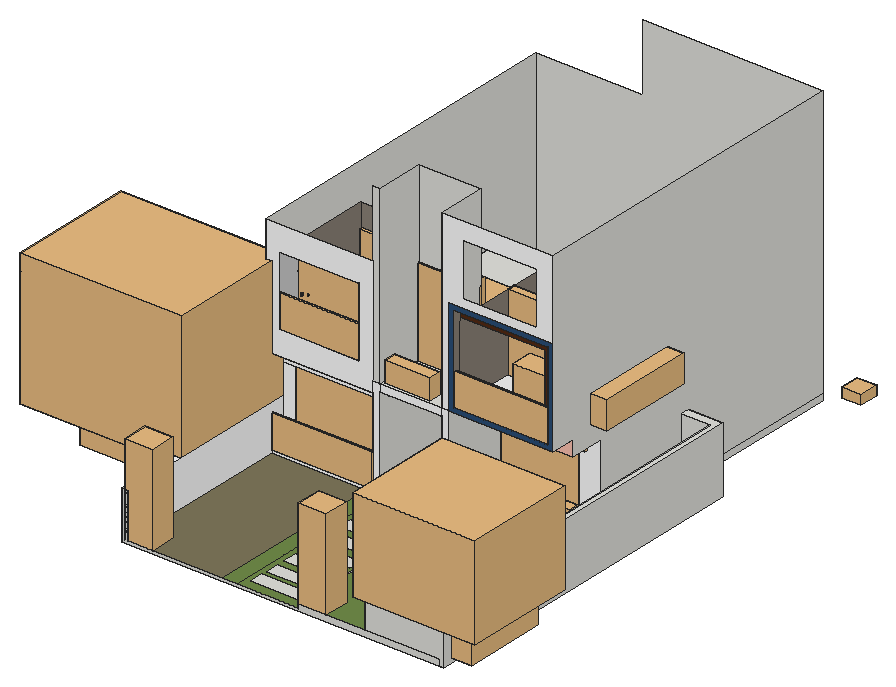
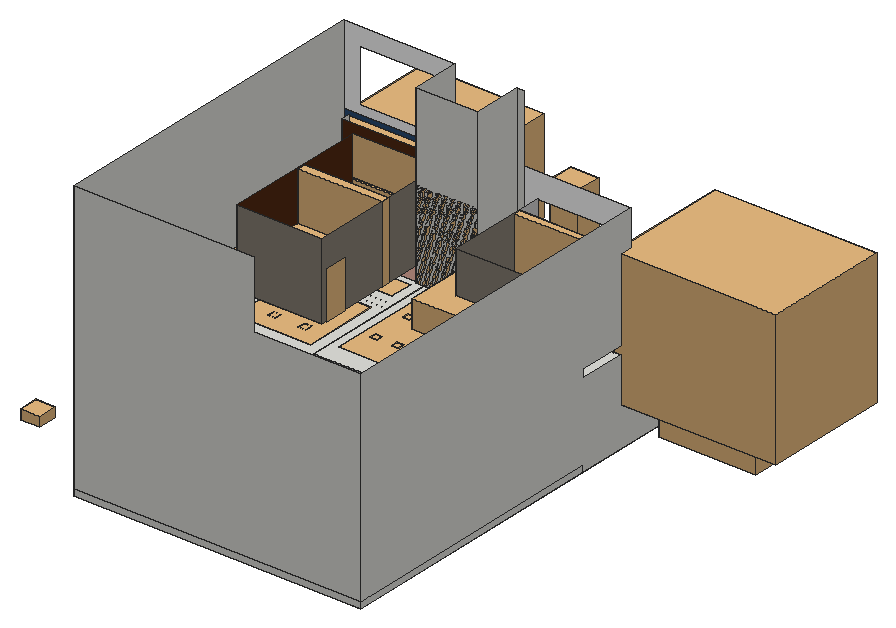
# SketchUp Ruby script. Lengths in inches.
U = 1.inch
M = Sketchup.active_model
def pt(a) = Geom::Point3d.new(a.map { |v| v * U })
def face(e, loops, mat)
  f = e.add_face(loops[0].map { |a| pt(a) })
  loops[1..].each { |l| e.add_face(l.map { |a| pt(a) }).erase! }
  f.material = f.back_material = mat if mat
  f
end
# faces: each face lists its corners as indices into pts; further lists are holes
def faces(e, pts, list, mat = nil) = list.each { |f| face(e, (f[0].is_a?(Array) ? f : [f]).map { |l| l.map { |i| pts[i] } }, mat) }
# xy, xz, yz: faces in a plane at the given z, y or x. An outline is a flat list of corners, or four numbers for a rectangle; further outlines are holes
def ring(l) = l.size == 4 ? [[l[0], l[1]], [l[2], l[1]], [l[2], l[3]], [l[0], l[3]]] : l.each_slice(2).to_a
def flat(e, list, mat, &to3) = list.each { |f| face(e, (f[0].is_a?(Array) ? f : [f]).map { |l| ring(l).map { |u, v| to3.(u, v) } }, mat) }
def xy(e, z, list, mat = nil) = flat(e, list, mat) { |x, y| [x, y, z] }
def xz(e, y, list, mat = nil) = flat(e, list, mat) { |x, z| [x, y, z] }
def yz(e, x, list, mat = nil) = flat(e, list, mat) { |y, z| [x, y, z] }
def lines(e, pts, list) = list.each { |a, b| e.add_line(pt(pts[a]), pt(pts[b])) }
# prism: a flat outline (further loops are holes) pulled along v
def prism(e, loops, v, mat = nil)
  f = face(e, loops, mat); d = Geom::Vector3d.new(v.map { |x| x * U })
  f.pushpull(f.normal.samedirection?(d) ? d.length : -d.length)
end
def box(e, o, s, mat = nil) = prism(e, [[o, [o[0] + s[0], o[1], o[2]], [o[0] + s[0], o[1] + s[1], o[2]], [o[0], o[1] + s[1], o[2]]]], [0, 0, s[2]], mat)
def at(x, y, z, deg = 0) = Geom::Transformation.translation(pt([x, y, z])) * Geom::Transformation.rotation(ORIGIN, Z_AXIS, deg.degrees)
def axes(o, x, y, z) = Geom::Transformation.new([*x, 0, *y, 0, *z, 0, *pt(o).to_a, 1])
def part(name) = M.definitions.add(name)
# library, detail: a bought-in or finely detailed component or shape, given as its bounding box
def library(name, o, s) = part(name).tap { |d| box(d.entities, o, s) }
def detail(e, o, s) = box(e.add_group.entities, o, s)
def put(e, d, t, mat = nil) = e.add_instance(d, t).tap { |i| i.material = mat if mat }
def group(e, t, mat = nil) = e.add_group.tap { |g| g.transformation = t; g.material = mat if mat }.entities
root = M.entities
M.materials.add("AM113_062_Tilia").color = [58, 81, 37]
M.materials.add("AM113_062_Tilia_Bark").color = [88, 85, 72]
M.materials.add("Concrete White 02 100cm").color = [209, 209, 209]
M.materials.add("Grass D 200cm").color = [112, 140, 73]
M.materials.add("Gravel E01 80cm").color = [127, 119, 91]
M.materials.add("Heather_Band").color = [140, 131, 120]
M.materials.add("Heather_PantShadow").color = [42, 79, 119]
M.materials.add("Tiles Marble Black 01 160cm").color = [31, 31, 31]
M.materials.add("Tiles Marble White 03 180cm").color = [241, 241, 241]
M.materials.add("Wall Paint White Semigloss 300cm").color = [255, 255, 255]
M.materials.add("Wood Mahogany 33-46 100cm").color = [83, 42, 20]
M.materials.add("[0131_Silver]").color = [192, 192, 192]
M.materials.add("[Color B01]").color = [255, 196, 178]
M.materials.add("efeu1").color = [18, 25, 13]
M.materials.add("efeu2").color = [43, 57, 29]
c1 = library("Lamp Outdoor 94-18",[-17.37,-12.57,0.01],[34.74,31.82,112.44])
c2 = library("skp108",[-1.77,-1.13,-0.05],[3.15,2.48,2.06])
c3 = library("skp10A",[-2.51,-1.55,0.73],[4.12,3.36,1.8])
c4 = part("tree")
put(c4.entities,c2,axes([-3.75,5.02,4.3],[-100,0,0],[0,100,0],[0,0,100]))
put(c4.entities,c3,axes([-24.21,-1.17,-13.42],[-100,0,0],[0,100,0],[0,0,100]))
c5 = library("Group\#39",[0,0,0],[56.8,25.91,35.15])
c6 = library("Rossi Sofa",[-52.17,-19.09,0],[104.34,38.18,34.45])
c7 = library("AM113_062_Tilia_Defintion",[-350.67,-364.73,-2.58],[672.29,726.36,1000])
c8 = library("AM113_062_Tilia_Defintion1",[-524.84,-500,219.37],[933.41,1000,877.77])
c9 = part("Group4\#1")
put(c9.entities,c7,axes([0,0,0],[0.28109,0,0],[0,0.28109,0],[0,0,0.28109]),"AM113_062_Tilia_Bark")
put(c9.entities,c8,axes([0,0,0],[0.33697,0,0],[0,0.33697,0],[0,0,0.33697]),"AM113_062_Tilia")
c10 = library("Group\#41",[0,0,0],[116.43,13.29,95.4])
c11 = library("My+Glass_Railing\#2",[-0.08,0,0],[125.4,2.52,40.9])
c12 = library("Entrance door assembly",[0,0,0],[51.57,9.61,84.84])
c13 = library("Dome Light",[-12,-12,0],[24,24,12])
c14 = part("Tlon Cubo 860 Ceiling 152 005")
xy(c14.entities,-3.04,[[-16.54,-16.54,-16.54,16.54,16.54,-16.54],[16.54,-16.54,-16.54,16.54,16.54,16.54]])
xy(c14.entities,0,[[-16.93,-16.93,16.93,-16.93,-16.93,16.93],[16.93,-16.93,16.93,16.93,-16.93,16.93]])
xz(c14.entities,-16.93,[[-16.93,-3.79,16.93,-3.79,-16.93,0],[16.93,-3.79,16.93,0,-16.93,0]])
xz(c14.entities,-16.3,[[-16.3,-3.66,-16.3,-3.24,16.3,-3.24],[-16.3,-3.66,16.3,-3.24,16.3,-3.66]])
xz(c14.entities,16.3,[[-16.3,-3.66,16.3,-3.24,-16.3,-3.24],[-16.3,-3.66,16.3,-3.66,16.3,-3.24]])
xz(c14.entities,16.93,[[-16.93,-3.79,-16.93,0,16.93,0],[-16.93,-3.79,16.93,0,16.93,-3.79]])
yz(c14.entities,-16.93,[[-16.93,-3.79,-16.93,0,16.93,0],[-16.93,-3.79,16.93,0,16.93,-3.79]])
yz(c14.entities,-16.3,[[-16.3,-3.66,16.3,-3.66,-16.3,-3.24],[16.3,-3.66,16.3,-3.24,-16.3,-3.24]])
yz(c14.entities,16.3,[[-16.3,-3.66,-16.3,-3.24,16.3,-3.66],[16.3,-3.66,-16.3,-3.24,16.3,-3.24]])
yz(c14.entities,16.93,[[-16.93,-3.79,16.93,-3.79,-16.93,0],[16.93,-3.79,16.93,0,-16.93,0]])
p = [[-16.93,-16.93,-3.79],[-16.93,16.93,-3.79],[-16.3,16.3,-3.66],[-16.3,-16.3,-3.66],[16.93,-16.93,-3.79],[16.3,-16.3,-3.66],
  [16.93,16.93,-3.79],[16.3,16.3,-3.66]]
faces(c14.entities,p,[[0,1,2],[2,3,0],[4,0,3],[3,5,4],[6,4,5],[5,7,6],[2,1,6],[6,7,2]])
c15 = library("Mesh Light\#3",[-0.5,-0.5,-0.1],[1,1,0.2])
c16 = library("Lamp Ceiling 114-44",[-1.26,-1.26,-3.9375],[2.52,2.52,3.9375])
c17 = library("Tlon Light 450 Ceiling 152 006",[-8.86,-8.86,-3.78],[17.72,17.72,3.56])
c18 = library("Group\#10",[-0.5,-0.5,-0.1],[94.5625,94.5625,0.2])
c19 = library("Group\#15",[-0.5,-0.5,-0.1],[105.0625,28.875,0.2])
c20 = library("Group\#9",[-0.5,-0.5,-0.1],[56.6875,175.375,0.2])
c21 = library("Planted timber trough",[0,0,0],[56.02,15.3,25.28])
c22 = library("Wall Panel 104-26",[-34.24,-2.8,0],[68.48,2.8,108.01])
c23 = library("Door 243 067",[-20.85,-3,0],[41.7,6,82.46])
c24 = library("BED_01",[-66.74,-61.37,0],[192.98,188.94,55.24])
c25 = library("My+Glass_Railing",[-0.08,0,0],[117.37,2.52,40.9])
c26 = library("My+Glass_Railing\#1",[-0.0625,0,0],[99.04,2.52,40.9])
c27 = part("ivyleaf_10")
p = [[0,0.5,-0.03],[-0.0625,2.02,-0.43],[-0.19,2.01,-0.46],[-0.54,1.05,-0.29],[-0.52,0.625,-0.18],[-0.83,0.76,-0.28],
  [-1.16,0.64,-0.33],[-1.15,0.33,-0.24],[-0.77,-0.39,0.02],[-0.3,-0.51,0.16],[0.04,-0.48,0.23],[-0.02,2.01,-0.4375],
  [-0.06,2.01,-0.43],[0.04,-0.49,0.23],[0.67,-0.49,0.14],[1.38,0.36,-0.2],[1.375,0.51,-0.24],[0.81,0.65,-0.19],
  [0.62,0.59,-0.15],[0.6,1.09,-0.28],[0.5,1.23,-0.31]]
faces(c27.entities,p,[[0,1,2,3,4,5,6,7,8,9,10],[11,12,0,13,14,15,16,17,18,19,20]],"efeu2")
c28 = part("ivyleaf_9")
p = [[1.54,2.16,1.25],[1.36,2.04,1.19],[-0.21,0.99,0.68],[-0.71,1.11,0.82],[-0.85,0.86,0.67],[-0.8,0.17,0.21],
  [-0.9,-0.01,0.1],[-0.67,-0.16,-0.02],[-0.08,-0.08,-0.05],[-0.03,-0.6,-0.4],[0.65,-0.88,-0.66],[0.83,-0.6,-0.49],
  [1.29,-0.42,-0.43],[1.8125,-0.07,-0.26],[1.21,0.44,0.15]]
faces(c28.entities,p,[[0,1,2,3,4,5,6,7,8,9,10,11,12,13,14]],"efeu1")
xy(root,-7.75,[[0,0,0,643.9375,356.8125,643.9375,356.8125,433.86,399.8125,433.86,399.8125,0]])
xy(root,-4.25,[[150.42,12.51,209.61,29.76],[150.42,36.64,209.61,53.89],[150.42,64.2,209.61,81.45],[150.42,92.51,209.61,109.76],[150.42,122.01,209.61,139.26],
  [150.42,150.82,209.61,168.07],[150.42,181.39,209.61,198.64]])
xy(root,-4.25,[[124.48,0,143.11,223.4375],[[143.11,0,219.21,223.4375],[150.42,181.39,209.61,198.64],[150.42,150.82,209.61,168.07],[150.42,122.01,209.61,139.26],[150.42,92.51,209.61,109.76],[150.42,64.2,209.61,81.45],[150.42,36.64,209.61,53.89],[150.42,12.51,209.61,29.76]]],"Grass D 200cm")
xy(root,-4.25,[[7.73,0,124.48,223.4375]],"Gravel E01 80cm")
xy(root,0,[[219.21,0,302.22,0,302.22,7.78,342.97,7.78,342.97,298,329.12,298,329.12,305.74,228.25,305.74,228.25,223.4375,219.21,223.4375],[342.97,7.78,393.4375,7.78,393.4375,422.3,356.8125,422.3,356.8125,298,342.97,298]],"Grass D 200cm")
xy(root,0,[[142.16,223.4375,219.21,442.3125]],"Tiles Marble Black 01 160cm")
xy(root,0,[[7.73,223.4375,133.125,223.4375,133.125,549.5625,24.6875,549.5625,24.6875,239.625,7.73,239.625],[228.25,305.74,354,453.5]],"Tiles Marble White 03 180cm")
xy(root,51.97,[[0,0,7.73,239.625]],"Wall Paint White Semigloss 300cm")
xy(root,74.875,[[302.22,0,399.8125,0,399.8125,433.86,356.8125,433.86,356.8125,422.3,393.4375,422.3,393.4375,7.78,302.22,7.78]])
xy(root,90.625,[[[24.6875,239.625,133.125,549.5625],[35.11,252,108.48,492.3125]],[37.11,254,106.48,490.3125]])
xy(root,97.625,[[0,239.625,133.125,298]])
xy(root,100.33,[[[228.25,254.1875,228.25,453.5,354,453.5,354,305.74,329.12,305.74,329.12,298,356.8125,298,356.8125,254.1875],[244.93,322.09,338.5,415.65],[243.03,262.87,347.1,290.75]],[245.03,264.87,345.1,288.75],[246.93,324.09,336.5,413.65]])
xy(root,107.3125,[[0,223.4375,133.125,298]])
xy(root,110.96,[[[142.16,223.4375,219.21,442.3125],[152.42,242.22,208.11,416.6]],[154.42,244.22,206.11,414.6]])
xy(root,120,[[142.16,223.4375,219.21,284.3125],[228.25,223.4375,356.8125,254.1875]])
xy(root,125.65,[[233.9,223.4375,351.16,233.25]])
xy(root,125.65,[[233.9,233.25,339.25,411.875]],"Tiles Marble White 03 180cm")
xy(root,137.04,[[17.04,223.4375,116.08,350]],"Tiles Marble White 03 180cm")
xz(root,0,[[0,-7.75,219.21,-7.75,219.21,-4.25,7.73,-4.25,7.73,51.97,0,51.97],[219.21,-7.75,393.4375,0],[393.4375,-7.75,399.8125,-7.75,399.8125,74.875,302.22,74.875,302.22,0,393.4375,0]])
xz(root,7.78,[[302.22,0,393.4375,74.875]])
xz(root,223.4375,[[133.125,120,142.16,337.75]])
xz(root,223.4375,[[[228.25,120,356.8125,240],[233.9,125.65,351.16,234.35]]],"Heather_PantShadow")
xz(root,223.4375,[[7.73,-4.25,219.21,-4.25,219.21,0,142.16,0,142.16,120,133.125,120,133.125,0,7.73,0],[219.21,0,228.25,120],[[0,107.3125,133.125,253.9375],[17.04,137.04,116.08,222.96]],[142.16,110.96,219.21,120],[[219.21,120,228.25,120,228.25,240,356.8125,240,356.8125,337.75,219.21,337.75],[245.01,250.82,337.3,316.43]]],"Wall Paint White Semigloss 300cm")
xz(root,233.25,[[339.25,125.65,351.16,125.65,351.16,234.35,233.9,234.35,233.9,222.44,339.25,222.44]],"Wood Mahogany 33-46 100cm")
xz(root,239.625,[[7.73,0,24.6875,0,24.6875,90.625,0,90.625,0,51.97,7.73,51.97],[0,90.625,133.125,97.625]],"Wall Paint White Semigloss 300cm")
xz(root,254.1875,[[228.25,100.33,356.8125,120]],"[Color B01]")
xz(root,284.3125,[[142.16,120,219.21,337.75]])
xz(root,298,[[0,97.625,133.125,107.3125]])
xz(root,298,[[329.12,0,356.8125,100.33]],"Wall Paint White Semigloss 300cm")
xz(root,305.74,[[329.12,0,354,100.33]])
xz(root,350,[[17.04,137.04,116.08,222.96]],"Heather_Band")
xz(root,411.875,[[233.9,125.65,339.25,220.38]],"Heather_Band")
xz(root,422.3,[[356.8125,0,393.4375,74.875]])
xz(root,433.86,[[356.8125,-7.75,399.8125,0],[356.8125,0,399.8125,74.875]])
xz(root,442.3125,[[142.16,0,219.21,110.96]])
xz(root,453.5,[[228.25,0,354,100.33]])
xz(root,549.5625,[[24.6875,0,133.125,90.625]],"[0131_Silver]")
xz(root,643.9375,[[0,-7.75,356.8125,0],[0,0,0,253.9375,133.125,253.9375,133.125,337.75,356.8125,337.75,356.8125,0]])
yz(root,0,[[0,-7.75,0,51.97,239.625,51.97,239.625,97.625,298,97.625,298,107.3125,223.4375,107.3125,223.4375,253.9375,643.9375,253.9375,643.9375,0,298,0,298,-7.75],[298,-7.75,643.9375,0]])
yz(root,7.73,[[0,-4.25,223.4375,-4.25,223.4375,0,239.625,0,239.625,51.97,0,51.97]],"Wall Paint White Semigloss 300cm")
yz(root,17.04,[[223.4375,137.04,251.4375,222.96]],"Concrete White 02 100cm")
yz(root,17.04,[[251.4375,137.04,350,222.96]],"Heather_Band")
yz(root,24.6875,[[239.625,0,549.5625,90.625]],"[0131_Silver]")
yz(root,116.08,[[223.4375,137.04,251.4375,222.96]],"Concrete White 02 100cm")
yz(root,116.08,[[251.4375,137.04,350,222.96]],"Heather_Band")
yz(root,133.125,[[223.4375,0,223.4375,107.3125,298,107.3125,298,97.625,239.625,97.625,239.625,90.625,549.5625,90.625,549.5625,0]],"[0131_Silver]")
yz(root,142.16,[[223.4375,0,442.3125,110.96],[223.4375,120,284.3125,337.75]])
yz(root,219.21,[[0,-4.25,223.4375,0],[223.4375,0,442.3125,110.96],[223.4375,120,284.3125,337.75]])
yz(root,228.25,[[223.4375,0,453.5,0,453.5,100.33,254.1875,100.33,254.1875,120,223.4375,120]])
yz(root,233.9,[[223.4375,125.65,233.25,234.35],[233.25,125.65,411.875,220.38]],"Heather_Band")
yz(root,302.22,[[0,0,7.78,74.875]])
yz(root,329.12,[[298,0,305.74,100.33]])
yz(root,339.25,[[233.25,125.65,411.875,220.38]],"Wood Mahogany 33-46 100cm")
yz(root,351.16,[[223.4375,125.65,233.25,234.35]])
yz(root,354,[[305.74,0,453.5,100.33]])
yz(root,356.8125,[[433.86,-7.75,643.9375,0],[298,0,422.3,0,422.3,74.875,433.86,74.875,433.86,0,643.9375,0,643.9375,337.75,223.4375,337.75,223.4375,120,254.1875,120,254.1875,100.33,298,100.33]])
yz(root,393.4375,[[7.78,0,422.3,74.875]])
yz(root,399.8125,[[0,-7.75,433.86,74.875]])
p = [[2465.46,-323.29,0],[2465.91,-323.26,0],[2465,-323.34,0],[2464.86,-323.37,0],[2466.37,-323.24,0],[2466.83,-323.23,0]]
lines(root,p,[[0,1],[2,0],[3,2],[4,5],[1,4]])
put(root,c1,at(20.83,12.57,-4.26))
put(root,c4,axes([362.14,56.04,-0.36],[0.37,0,0],[0,0.415,0],[0,0,0.645]))
put(root,c5,axes([280.125,285.58,-0.06],[0.855,0,0],[0,0.5,0],[0,0,0.5]))
put(root,c5,axes([232.875,285.58,-0.06],[0.855,0,0],[0,0.5,0],[0,0,0.5]))
put(root,c1,at(236.59,12.57,-0.01))
put(root,c6,at(60.44,371.51,0,89.1))
put(root,c9,axes([-79.97,161.19,0.41],[0.637,0,0],[0,0.4655,0],[0,0,0.567]))
put(root,c10,axes([24.6875,239.625,0],[0.93134,0,0],[0,0.76551,0],[0,0,0.95072]))
put(root,c11,at(7.81,222.57,0.2))
put(root,c12,at(204.875,442.3125,2.4375,180))
put(root,c10,axes([228.25,303.72,5.5625],[0.90367,0,0],[0,0.76551,0],[0,0,0.99334]))
put(root,c13,at(429.59,608.66,37.4375))
put(root,c14,axes([50.28,320.87,90.625],[0.2697,0,0],[0,0.2697,0],[0,0,0.2697]))
put(root,c14,axes([87.9,320.87,90.625],[0.2697,0,0],[0,0.2697,0],[0,0,0.2697]))
put(root,c14,axes([87.9,269.25,90.625],[0.2697,0,0],[0,0.2697,0],[0,0,0.2697]))
put(root,c14,axes([50.28,269.25,90.625],[0.2697,0,0],[0,0.2697,0],[0,0,0.2697]))
put(root,c14,axes([50.28,421.18,90.625],[0.2697,0,0],[0,0.2697,0],[0,0,0.2697]))
put(root,c14,axes([87.9,369.56,90.625],[0.2697,0,0],[0,0.2697,0],[0,0,0.2697]))
put(root,c14,axes([87.9,421.18,90.625],[0.2697,0,0],[0,0.2697,0],[0,0,0.2697]))
put(root,c14,axes([50.28,369.56,90.625],[0.2697,0,0],[0,0.2697,0],[0,0,0.2697]))
g1 = group(root,at(35.11,252,90.625))
xy(g1,0,[[[0,0,73.375,240.3125],[2,2,71.375,238.3125]]])
put(g1,c15,axes([36.6875,120.16,0],[74.375,0,0],[0,241.3125,0],[0,0,1]))
put(root,c16,at(353.99,277.26,100.41))
put(root,c17,axes([314.64,278.625,100.43],[0.462,0,0],[0,0.462,0],[0,0,0.462]))
put(root,c17,axes([267,278.93,100.43],[0.462,0,0],[0,0.462,0],[0,0,0.462]))
put(root,c14,axes([308.71,339.98,100.33],[0.2697,0,0],[0,0.2697,0],[0,0,0.2697]))
put(root,c14,axes([271.09,339.98,100.33],[0.2697,0,0],[0,0.2697,0],[0,0,0.2697]))
put(root,c14,axes([271.09,391.61,100.33],[0.2697,0,0],[0,0.2697,0],[0,0,0.2697]))
put(root,c14,axes([308.71,391.61,100.33],[0.2697,0,0],[0,0.2697,0],[0,0,0.2697]))
put(root,c18,at(244.93,322.09,100.33))
put(root,c19,at(243.03,262.87,100.33))
put(root,c16,at(212.06,229.89,110.96))
put(root,c16,at(149.87,229.89,110.96))
put(root,c17,axes([192.38,276.25,111.2],[0.462,0,0],[0,0.462,0],[0,0,0.462]))
put(root,c17,axes([165.75,276.25,111.2],[0.462,0,0],[0,0.462,0],[0,0,0.462]))
put(root,c17,axes([165.75,379.0625,111.2],[0.462,0,0],[0,0.462,0],[0,0,0.462]))
put(root,c17,axes([192.38,379.0625,111.2],[0.462,0,0],[0,0.462,0],[0,0,0.462]))
put(root,c17,axes([165.75,328.5,111.2],[0.462,0,0],[0,0.462,0],[0,0,0.462]))
put(root,c17,axes([192.38,328.5,111.2],[0.462,0,0],[0,0.462,0],[0,0,0.462]))
put(root,c20,at(152.42,242.22,110.96))
put(root,c21,at(144.5,227.77,120))
put(root,c22,axes([180.6875,284.3125,120],[1.1252,0,0],[0,0.99999,0],[0,0,1.01605]))
put(root,c23,axes([235.22,391.04,125],[0,0.68565,0],[-0.71,0,0],[0,0,0.71]))
put(root,c24,axes([299.26,358.8125,125.35],[0,-0.62,0],[0.62,0,0],[0,0,0.62]))
put(root,c10,axes([233.35,307.68,125.65],[0.90367,0,0],[0,0.76551,0],[0,0,0.99334]))
put(root,c25,at(233.875,223.4375,125.65))
put(root,c5,axes([235.86,225.56,126.78],[0.855,0,0],[0,0.5,0],[0,0,0.5]))
put(root,c5,axes([283.11,225.56,126.78],[0.855,0,0],[0,0.5,0],[0,0,0.5]))
put(root,c23,axes([33.12,349,137.01],[0.68565,0,0],[0,0.71,0],[0,0,0.71]))
put(root,c5,axes([16.73,225.56,137.03],[0.855,0,0],[0,0.5,0],[0,0,0.5]))
put(root,c5,axes([63.98,225.56,137.03],[0.855,0,0],[0,0.5,0],[0,0,0.5]))
put(root,c26,at(17.11,223.42,137.04))
put(root,c10,axes([17.03,251.43,137.04],[0.85079,0,0],[0,0.65068,0],[0,0,0.90061]))
put(root,c24,axes([82.57,317.85,137.04],[0.5022,0,0],[0,0.5022,0],[0,0,0.62273]))
put(root,c27,axes([46.51,222.03,186.16],[0.20024,-0.20938,-0.40751],[-0.27899,0.29704,-0.28971],[0.36341,0.34341,0.00212]))
put(root,c27,axes([46.59,222.03,186.78],[-0.45429,0.10663,-0.17958],[0.17244,-0.05104,-0.46654],[-0.11783,-0.48582,0.0096]))
put(root,c27,axes([46.89,220.16,186.86],[-0.05714,-0.42724,0.25338],[0.16718,-0.25671,-0.39516],[0.46775,0.03956,0.17219]))
put(root,c28,axes([47.13,220.47,187.03],[-0.05543,-0.49268,0.06475],[0.16254,-0.07954,-0.46611],[0.46958,-0.03062,0.16897]))
put(root,c27,axes([47.28,220.93,187.02],[0.07629,-0.21786,0.44353],[0.12255,-0.42642,-0.23054],[0.47871,0.14388,-0.01167]))
put(root,c27,axes([46.23,222,186.47],[0.37486,-0.30699,0.12344],[-0.08863,0.08656,0.48441],[-0.31879,-0.38505,0.01048]))
put(root,c27,axes([46.59,222.07,187.64],[-0.1208,-0.47136,0.11501],[-0.01977,-0.11364,-0.48651],[0.48479,-0.12208,0.00882]))
put(root,c28,axes([53.32,223.1875,187.65],[-0.0629,0.15764,0.47031],[-0.19548,0.42783,-0.16955],[-0.45588,-0.20521,0.00781]))
put(root,c27,axes([46.19,221.875,188.25],[0.33976,-0.08092,-0.35779],[-0.34085,0.11062,-0.34869],[0.13559,0.48085,0.02]))
put(root,c28,axes([46.5,222.05,188.38],[0.14,-0.41353,0.2437],[0.07912,-0.2305,-0.43659],[0.47343,0.16081,0.0009]))
